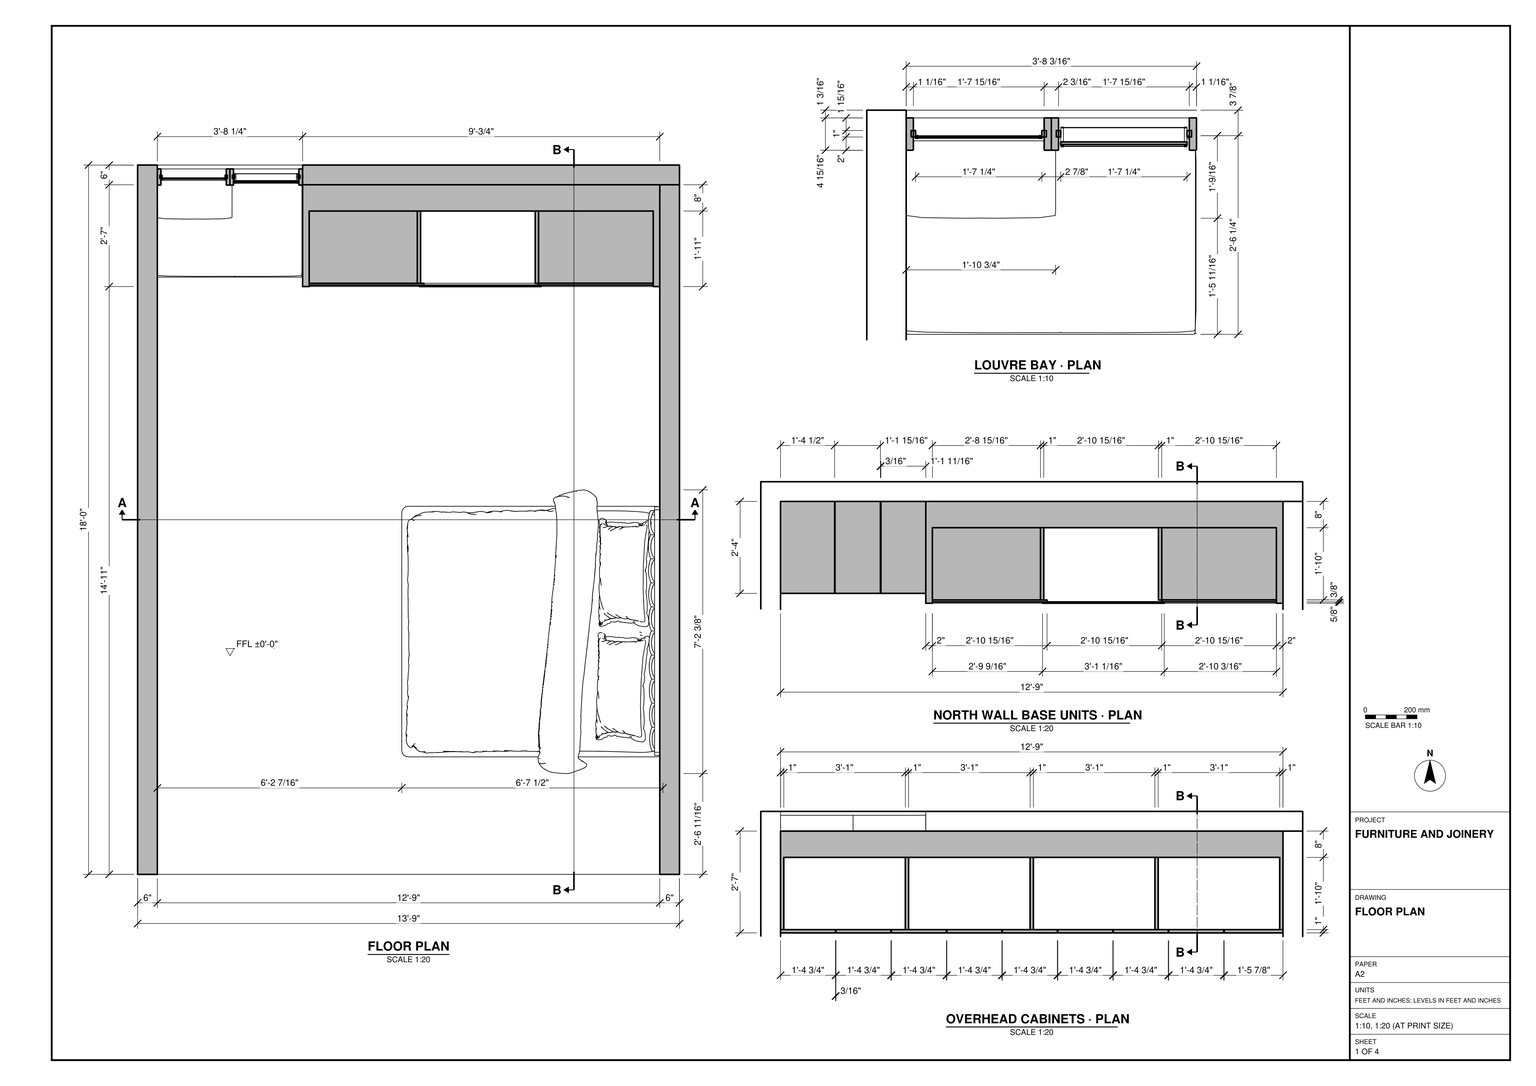
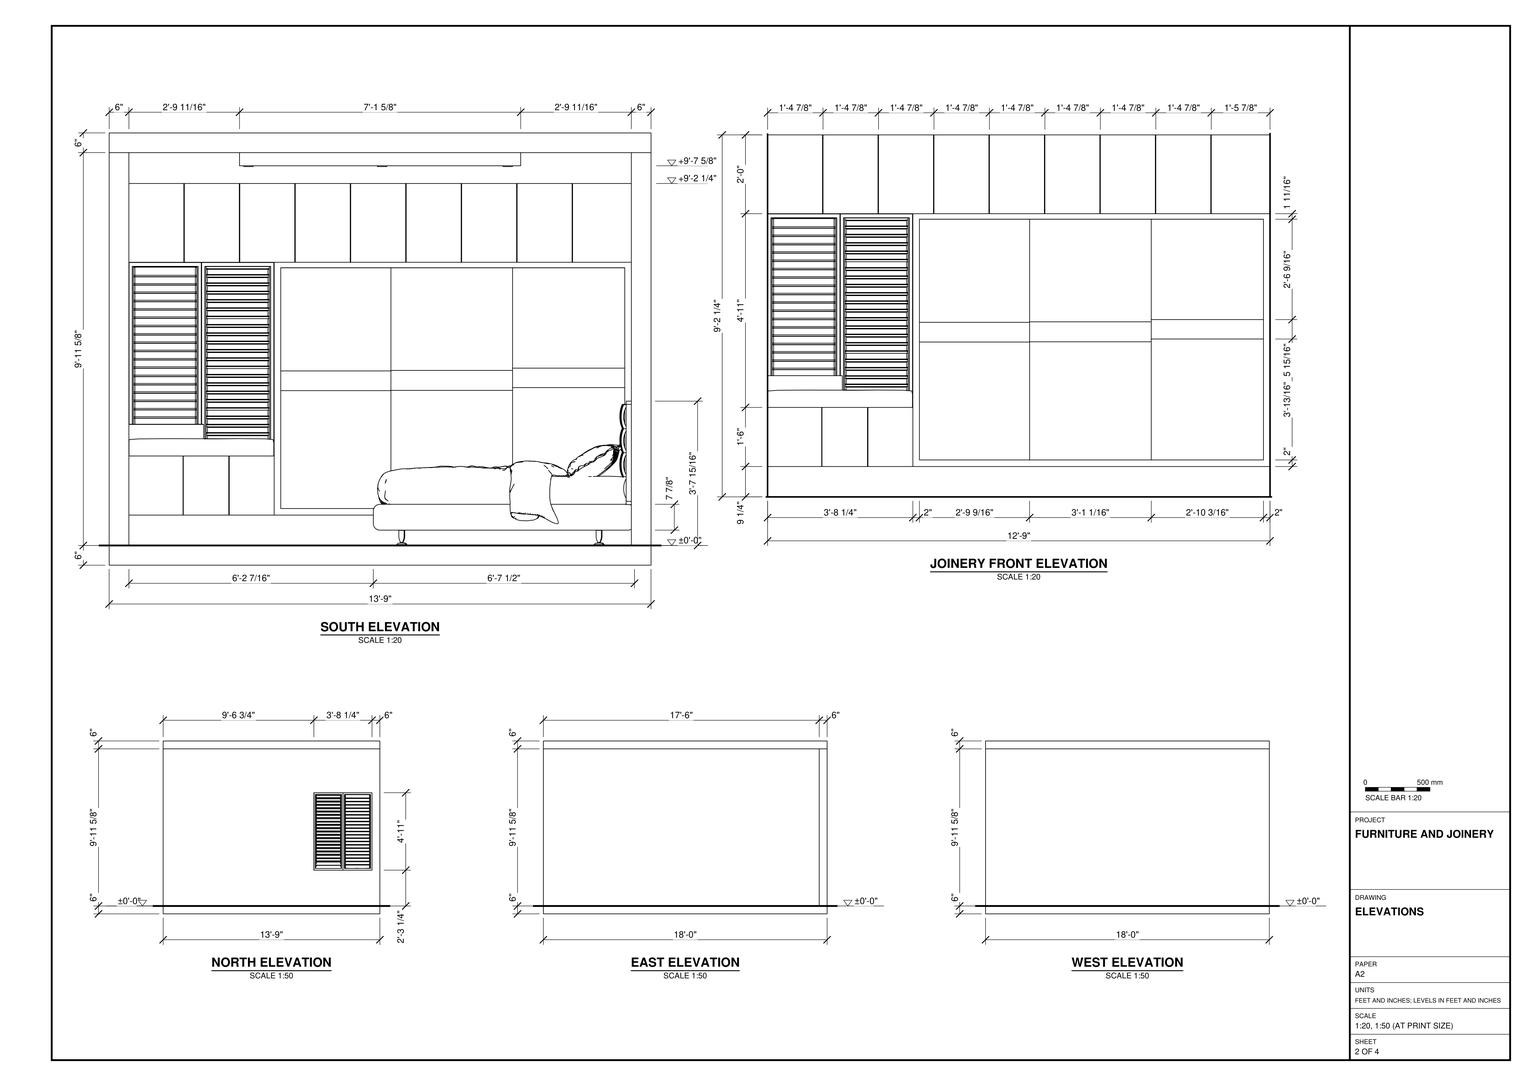
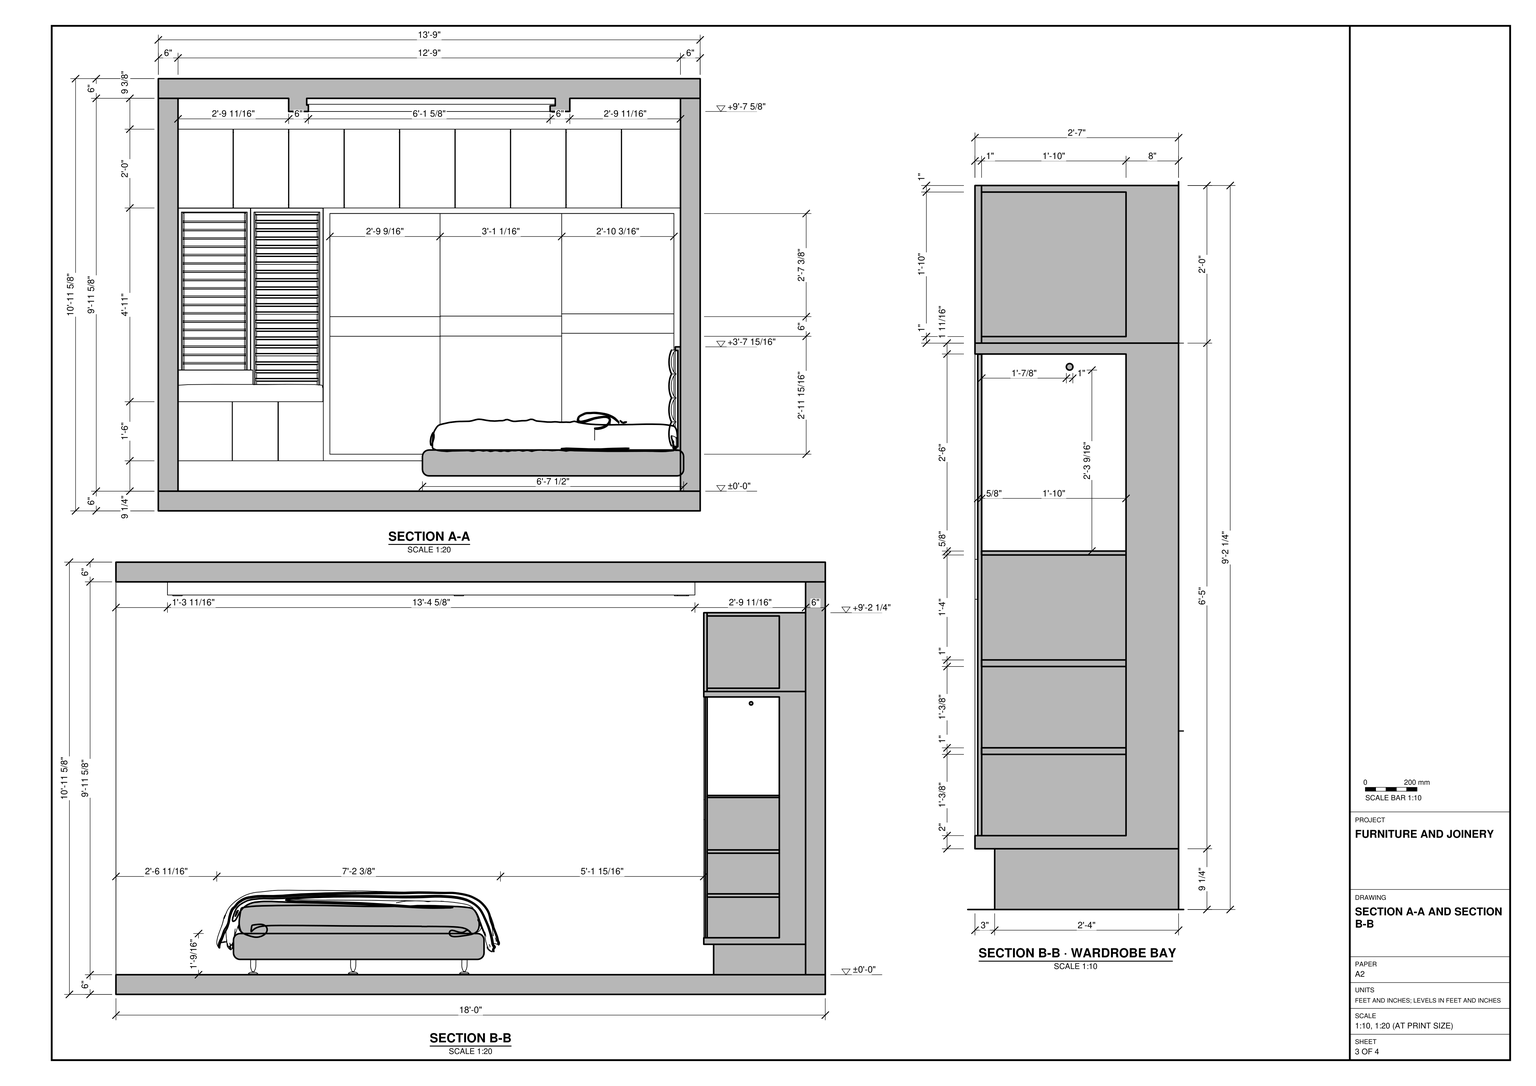
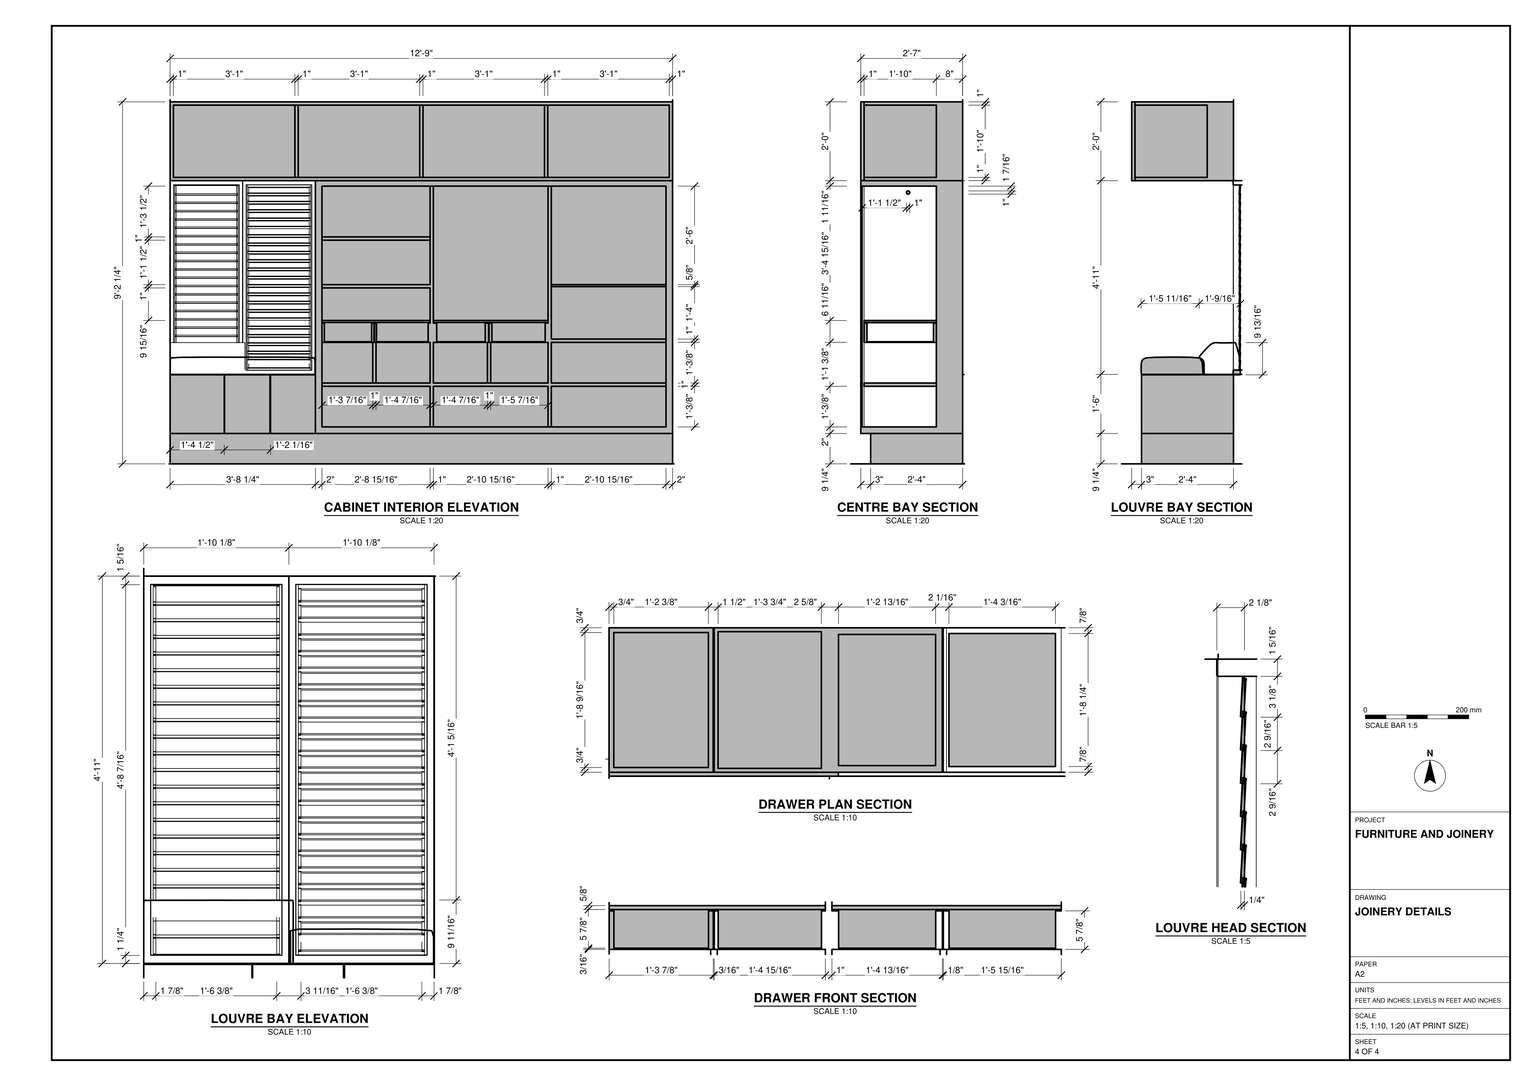
Model the bedroom in SketchUp using task_files/diagram_01.pdf. Work in feet and inches. Set the finished floor level to ±0'-0". The room shell measures 13'-9" east to west, 18'-0" north to south and 10'-11 5/8" high overall. Model the 6" side and north walls between the floor and ceiling slabs. Leave the south end open as drawn, and include the elongated ceiling feature shown in the sections.

Fit the joinery across the north wall. At the west end, place the two framed louvred window units above the sill and low cabinets. Beside them, model the three tall wardrobe bays with the front divisions shown in elevation. Use the wardrobe section to set out the recessed plinth, shelves and hanging rail. Continue the overhead cabinets across both the window bay and the wardrobes. Place the bed with its headboard against the east wall and its foot facing west, leaving the clearances shown in plan. Include the raised bed base, mattress and bedding.

Decor and loose items may be any suitable library components. Keep shell elements and each furniture or joinery piece in separate groups or components, and use components for repeated parts. Save one SketchUp model as output_files/bedroom_with_fitted_wardrobes_and_a_louvred_window.skp.

# SketchUp Ruby script. Lengths in inches.
U = 1.inch
M = Sketchup.active_model
def pt(a) = Geom::Point3d.new(a.map { |v| v * U })
def face(e, loops, mat)
  f = e.add_face(loops[0].map { |a| pt(a) })
  loops[1..].each { |l| e.add_face(l.map { |a| pt(a) }).erase! }
  f.material = f.back_material = mat if mat
  f
end
# faces: each face lists its corners as indices into pts; further lists are holes
def faces(e, pts, list, mat = nil) = list.each { |f| face(e, (f[0].is_a?(Array) ? f : [f]).map { |l| l.map { |i| pts[i] } }, mat) }
# xy, xz, yz: faces in a plane at the given z, y or x. An outline is a flat list of corners, or four numbers for a rectangle; further outlines are holes
def ring(l) = l.size == 4 ? [[l[0], l[1]], [l[2], l[1]], [l[2], l[3]], [l[0], l[3]]] : l.each_slice(2).to_a
def flat(e, list, mat, &to3) = list.each { |f| face(e, (f[0].is_a?(Array) ? f : [f]).map { |l| ring(l).map { |u, v| to3.(u, v) } }, mat) }
def xy(e, z, list, mat = nil) = flat(e, list, mat) { |x, y| [x, y, z] }
def xz(e, y, list, mat = nil) = flat(e, list, mat) { |x, z| [x, y, z] }
def yz(e, x, list, mat = nil) = flat(e, list, mat) { |y, z| [x, y, z] }
def lines(e, pts, list) = list.each { |a, b| e.add_line(pt(pts[a]), pt(pts[b])) }
# prism: a flat outline (further loops are holes) pulled along v
def prism(e, loops, v, mat = nil)
  f = face(e, loops, mat); d = Geom::Vector3d.new(v.map { |x| x * U })
  f.pushpull(f.normal.samedirection?(d) ? d.length : -d.length)
end
def box(e, o, s, mat = nil) = prism(e, [[o, [o[0] + s[0], o[1], o[2]], [o[0] + s[0], o[1] + s[1], o[2]], [o[0], o[1] + s[1], o[2]]]], [0, 0, s[2]], mat)
def at(x, y, z, deg = 0) = Geom::Transformation.translation(pt([x, y, z])) * Geom::Transformation.rotation(ORIGIN, Z_AXIS, deg.degrees)
def axes(o, x, y, z) = Geom::Transformation.new([*x, 0, *y, 0, *z, 0, *pt(o).to_a, 1])
def part(name) = M.definitions.add(name)
# library, detail: a bought-in or finely detailed component or shape, given as its bounding box
def library(name, o, s) = part(name).tap { |d| box(d.entities, o, s) }
def detail(e, o, s) = box(e.add_group.entities, o, s)
def put(e, d, t, mat = nil) = e.add_instance(d, t).tap { |i| i.material = mat if mat }
def group(e, t, mat = nil) = e.add_group.tap { |g| g.transformation = t; g.material = mat if mat }.entities
root = M.entities
M.materials.add("GLASS BLADE REFRACTION").color = [24, 24, 24]
M.materials["GLASS BLADE REFRACTION"].alpha = 0.5
M.materials.add("JalousieFrame").color = [89, 86, 86]
M.materials.add("[0002_MediumVioletRed]").color = [204, 196, 185]
M.materials.add("[0003_DeepPink]").color = [255, 20, 147]
M.materials.add("[Color A01]").color = [207, 198, 188]
M.materials.add("[Color A01]1").color = [135, 122, 106]
M.materials.add("[Color A01]2").color = [96, 100, 74]
M.materials.add("[Color A02]").color = [146, 166, 154]
M.materials.add("[Color A02]1").color = [177, 163, 128]
M.materials.add("[Color A03]").color = [255, 101, 101]
M.materials.add("[Color H05]").color = [0, 255, 255]
M.materials.add("[Color M00]").color = [255, 255, 255]
M.materials.add("[Metal Corrugated Shiny]").color = [193, 193, 193]
M.materials.add("[Tile Large Brown]").color = [195, 178, 159]
M.materials.add("[Translucent Glass Blue]").color = [100, 149, 237]
M.materials["[Translucent Glass Blue]"].alpha = 0.5
M.materials.add("[Translucent Glass Corrugated]").color = [141, 158, 145]
M.materials["[Translucent Glass Corrugated]"].alpha = 0.8
M.materials.add("[Translucent_Glass_Blue]1").color = [0, 0, 0]
M.materials["[Translucent_Glass_Blue]1"].alpha = 0
M.materials.add("[Wood OSB]").color = [240, 195, 122]
c1 = part("Louvre end clip")
prism(c1.entities,[[[0,0.74,4.2],[0,0.38,4.24],[0,-0.06,-0.03],[0,0.29,-0.06],[0,0.3125,0.17],[0,0.26,0.18],[0,0.24,-0.02],[0,-0.02,0.01],[0,0.42,4.2],[0,0.68,4.17],[0,0.66,3.97],[0,0.71,3.97]]],[-0.59,0,0],"JalousieFrame")
c2 = part("Louvre blade")
xy(c2.entities,0,[[3.2,0,48.34,0.24]],"GLASS BLADE REFRACTION")
xy(c2.entities,4.17,[[3.2,0,48.34,0.24]],"GLASS BLADE REFRACTION")
xz(c2.entities,0,[[3.2,0,48.34,4.17]],"[Translucent Glass Blue]")
xz(c2.entities,0.24,[[3.2,0,48.34,4.17]],"[Translucent_Glass_Blue]1")
yz(c2.entities,3.2,[[0,0,0.24,4.17]],"[Translucent_Glass_Blue]1")
yz(c2.entities,48.34,[[0,0,0.24,4.17]],"[Translucent_Glass_Blue]1")
c3 = part("Louvre blade assembly")
put(c3.entities,c1,axes([29.56,0.12,0.28],[1,0,0],[0,1.01433,-0.13582],[0,-0.20296,0.86161]))
put(c3.entities,c1,axes([1.96,0.12,0.28],[-1,0,0],[0,1.01433,-0.13582],[0,-0.20296,0.86161]))
put(c3.entities,c2,axes([0,0.12,0.3],[0.61176,0,0],[0,1.02999,-0.22514],[0,-0.09582,0.84269]))
c4 = part("Louvre blade assembly \#1")
put(c4.entities,c3,axes([-2.4,1.66,-0.39],[1.63462,0,0],[0,0.98741,-0.15853],[0,0.15779,0.98741]),"[Translucent Glass Corrugated]")
c5 = part("Group6\#2")
box(c5.entities,[-2.07,2.02,1.67],[0.98,0.98,67.72],"JalousieFrame")
c6 = part("Louvred window")
xz(c6.entities,3.09,[[2.06,1.67,29.07,69.26]])
put(c6.entities,c4,axes([1.57,0.98,65.83],[0.61176,0,0],[0,1,0],[0,0,0.99766]))
put(c6.entities,c4,axes([1.57,0.98,62.79],[0.61176,0,0],[0,1,0],[0,0,0.99766]))
put(c6.entities,c4,axes([1.57,0.98,59.75],[0.61176,0,0],[0,1,0],[0,0,0.99766]))
put(c6.entities,c4,axes([1.57,0.98,56.7],[0.61176,0,0],[0,1,0],[0,0,0.99766]))
put(c6.entities,c4,axes([1.57,0.98,53.66],[0.61176,0,0],[0,1,0],[0,0,0.99766]))
put(c6.entities,c4,axes([1.57,0.98,50.61],[0.61176,0,0],[0,1,0],[0,0,0.99766]))
put(c6.entities,c4,axes([1.57,0.98,47.57],[0.61176,0,0],[0,1,0],[0,0,0.99766]))
put(c6.entities,c4,axes([1.57,0.98,44.53],[0.61176,0,0],[0,1,0],[0,0,0.99766]))
put(c6.entities,c4,axes([1.57,0.98,41.48],[0.61176,0,0],[0,1,0],[0,0,0.99766]))
put(c6.entities,c4,axes([1.57,0.98,38.4375],[0.61176,0,0],[0,1,0],[0,0,0.99766]))
put(c6.entities,c4,axes([1.57,0.98,35.39],[0.61176,0,0],[0,1,0],[0,0,0.99766]))
put(c6.entities,c4,axes([1.57,0.98,32.35],[0.61176,0,0],[0,1,0],[0,0,0.99766]))
put(c6.entities,c4,axes([1.57,0.98,29.31],[0.61176,0,0],[0,1,0],[0,0,0.99766]))
put(c6.entities,c4,axes([1.57,0.98,26.26],[0.61176,0,0],[0,1,0],[0,0,0.99766]))
put(c6.entities,c4,axes([1.57,0.98,23.22],[0.61176,0,0],[0,1,0],[0,0,0.99766]))
put(c6.entities,c4,axes([1.57,0.98,20.17],[0.61176,0,0],[0,1,0],[0,0,0.99766]))
put(c6.entities,c4,axes([1.57,0.98,17.13],[0.61176,0,0],[0,1,0],[0,0,0.99766]))
put(c6.entities,c4,axes([1.57,0.98,14.09],[0.61176,0,0],[0,1,0],[0,0,0.99766]))
put(c6.entities,c4,axes([1.57,0.98,11.04],[0.61176,0,0],[0,1,0],[0,0,0.99766]))
put(c6.entities,c4,axes([1.57,0.98,8],[0.61176,0,0],[0,1,0],[0,0,0.99766]))
put(c6.entities,c4,axes([1.57,0.98,4.95],[0.61176,0,0],[0,1,0],[0,0,0.99766]))
put(c6.entities,c4,axes([1.57,0.98,1.91],[0.61176,0,0],[0,1,0],[0,0,0.99766]))
g1 = group(c6.entities,at(0,0.98,0.1))
xy(g1,0,[[0,0.1,31.72,4.92]],"JalousieFrame")
xy(g1,1.57,[[1.57,0.1,30.15,4.92]],"JalousieFrame")
xy(g1,69.29,[[1.57,0.1,30.15,4.92]],"JalousieFrame")
xy(g1,70.87,[[0,0.1,31.72,4.92]],"JalousieFrame")
xz(g1,0,[[[0.1,0.1,31.625,70.77],[1.47,1.48,30.25,69.39]]],"JalousieFrame")
xz(g1,4.92,[[[0,0,31.72,70.87],[1.57,1.57,30.15,69.29]]],"JalousieFrame")
yz(g1,0,[[0.1,0,4.92,70.87]],"JalousieFrame")
yz(g1,1.57,[[0.1,1.57,4.92,69.29]],"JalousieFrame")
yz(g1,30.15,[[0.1,1.57,4.92,69.29]],"JalousieFrame")
yz(g1,31.72,[[0.1,0,4.92,70.87]],"JalousieFrame")
p = [[0,0.1,70.87],[0,0.1,0],[0.1,0,0.1],[0.1,0,70.77],[31.72,0.1,0],[31.625,0,0.1],
  [31.72,0.1,70.87],[31.625,0,70.77],[30.15,0.1,1.57],[1.57,0.1,1.57],[1.47,0,1.48],[30.25,0,1.48],
  [1.57,0.1,69.29],[1.47,0,69.39],[30.15,0.1,69.29],[30.25,0,69.39]]
faces(g1,p,[[0,1,2,3],[1,4,5,2],[4,6,7,5],[8,9,10,11],[9,12,13,10],[14,8,11,15],[12,14,15,13],[6,0,3,7]],"JalousieFrame")
put(c6.entities,c5,axes([31.72,0.98,0],[0.99482,0,0],[0,1,0],[0,0,1]))
put(c6.entities,c5,axes([0,0.98,0],[-0.99482,0,0],[0,1,0],[0,0,1]))
c7 = part("Louvre blade assembly \#2")
put(c7.entities,c3,axes([-2.4,0.24,0.625],[1.63462,0,0],[0,0.5,-0.86805],[0,0.864,0.5]))
c8 = part("Group6\#1")
box(c8.entities,[-2.07,2.02,1.67],[0.98,0.98,67.72],"JalousieFrame")
c9 = part("Louvred window \#1")
put(c9.entities,c7,axes([1.57,0.98,65.83],[0.61176,0,0],[0,1,0],[0,0,0.99766]))
put(c9.entities,c7,axes([1.57,0.98,62.79],[0.61176,0,0],[0,1,0],[0,0,0.99766]))
put(c9.entities,c7,axes([1.57,0.98,59.75],[0.61176,0,0],[0,1,0],[0,0,0.99766]))
put(c9.entities,c7,axes([1.57,0.98,56.7],[0.61176,0,0],[0,1,0],[0,0,0.99766]))
put(c9.entities,c7,axes([1.57,0.98,53.66],[0.61176,0,0],[0,1,0],[0,0,0.99766]))
put(c9.entities,c7,axes([1.57,0.98,50.61],[0.61176,0,0],[0,1,0],[0,0,0.99766]))
put(c9.entities,c7,axes([1.57,0.98,47.57],[0.61176,0,0],[0,1,0],[0,0,0.99766]))
put(c9.entities,c7,axes([1.57,0.98,44.53],[0.61176,0,0],[0,1,0],[0,0,0.99766]))
put(c9.entities,c7,axes([1.57,0.98,41.48],[0.61176,0,0],[0,1,0],[0,0,0.99766]))
put(c9.entities,c7,axes([1.57,0.98,38.4375],[0.61176,0,0],[0,1,0],[0,0,0.99766]))
put(c9.entities,c7,axes([1.57,0.98,35.39],[0.61176,0,0],[0,1,0],[0,0,0.99766]))
put(c9.entities,c7,axes([1.57,0.98,32.35],[0.61176,0,0],[0,1,0],[0,0,0.99766]))
put(c9.entities,c7,axes([1.57,0.98,29.31],[0.61176,0,0],[0,1,0],[0,0,0.99766]))
put(c9.entities,c7,axes([1.57,0.98,26.26],[0.61176,0,0],[0,1,0],[0,0,0.99766]))
put(c9.entities,c7,axes([1.57,0.98,23.22],[0.61176,0,0],[0,1,0],[0,0,0.99766]))
put(c9.entities,c7,axes([1.57,0.98,20.17],[0.61176,0,0],[0,1,0],[0,0,0.99766]))
put(c9.entities,c7,axes([1.57,0.98,17.13],[0.61176,0,0],[0,1,0],[0,0,0.99766]))
put(c9.entities,c7,axes([1.57,0.98,14.09],[0.61176,0,0],[0,1,0],[0,0,0.99766]))
put(c9.entities,c7,axes([1.57,0.98,11.04],[0.61176,0,0],[0,1,0],[0,0,0.99766]))
put(c9.entities,c7,axes([1.57,0.98,8],[0.61176,0,0],[0,1,0],[0,0,0.99766]))
put(c9.entities,c7,axes([1.57,0.98,4.95],[0.61176,0,0],[0,1,0],[0,0,0.99766]))
put(c9.entities,c7,axes([1.57,0.98,1.91],[0.61176,0,0],[0,1,0],[0,0,0.99766]))
g2 = group(c9.entities,at(0,0.98,0.1))
xy(g2,0,[[0,0.1,31.72,4.92]],"JalousieFrame")
xy(g2,1.57,[[1.57,0.1,30.15,4.92]],"JalousieFrame")
xy(g2,69.29,[[1.57,0.1,30.15,4.92]],"JalousieFrame")
xy(g2,70.87,[[0,0.1,31.72,4.92]],"JalousieFrame")
xz(g2,0,[[[0.1,0.1,31.625,70.77],[1.47,1.48,30.25,69.39]]],"JalousieFrame")
xz(g2,4.92,[[[0,0,31.72,70.87],[1.57,1.57,30.15,69.29]]],"JalousieFrame")
yz(g2,0,[[0.1,0,4.92,70.87]],"JalousieFrame")
yz(g2,1.57,[[0.1,1.57,4.92,69.29]],"JalousieFrame")
yz(g2,30.15,[[0.1,1.57,4.92,69.29]],"JalousieFrame")
yz(g2,31.72,[[0.1,0,4.92,70.87]],"JalousieFrame")
p = [[0,0.1,70.87],[0,0.1,0],[0.1,0,0.1],[0.1,0,70.77],[31.72,0.1,0],[31.625,0,0.1],
  [31.72,0.1,70.87],[31.625,0,70.77],[30.15,0.1,1.57],[1.57,0.1,1.57],[1.47,0,1.48],[30.25,0,1.48],
  [1.57,0.1,69.29],[1.47,0,69.39],[30.15,0.1,69.29],[30.25,0,69.39]]
faces(g2,p,[[0,1,2,3],[1,4,5,2],[4,6,7,5],[8,9,10,11],[9,12,13,10],[14,8,11,15],[12,14,15,13],[6,0,3,7]],"JalousieFrame")
put(c9.entities,c8,axes([31.72,0.98,0],[0.99482,0,0],[0,1,0],[0,0,1]))
put(c9.entities,c8,axes([0,0.98,0],[-0.99482,0,0],[0,1,0],[0,0,1]))
c10 = part("JSilva Jalousie")
put(c10.entities,c6,axes([-10.84,-0.98,0.02],[-0.66344,0,0],[0,1,0],[0,0,0.83238]))
put(c10.entities,c9,axes([10.2,-0.98,0.02],[-0.66344,0,0],[0,1,0],[0,0,0.83238]))
c11 = library("Natuzzi-Forma-2818-373",[-24.875,-9.99,1.67],[57.88,39.07,27.9])
c12 = part("Round vent grille")
xy(c12.entities,-0.25,[[[1.4375,0,1.07,0.05,0.72,0.19,0.42,0.42,0.19,0.72,0.05,1.07,0,1.4375,0.05,1.81,0.19,2.16,0.42,2.45,0.72,2.68,1.07,2.83,1.4375,2.875,1.81,2.83,2.16,2.68,2.45,2.45,2.68,2.16,2.83,1.81,2.875,1.4375,2.83,1.07,2.68,0.72,2.45,0.42,2.16,0.19,1.81,0.05],[1.4375,0.47,1.6875,0.51,1.92,0.6,2.12,0.76,2.27,0.96,2.37,1.1875,2.4,1.4375,2.37,1.6875,2.27,1.92,2.12,2.12,1.92,2.27,1.6875,2.37,1.4375,2.4,1.1875,2.37,0.96,2.27,0.76,2.12,0.6,1.92,0.51,1.6875,0.47,1.4375,0.51,1.1875,0.6,0.96,0.76,0.76,0.96,0.6,1.1875,0.51]]])
xy(c12.entities,-0.0625,[[1.4375,0.47,1.1875,0.51,0.96,0.6,0.76,0.76,0.6,0.96,0.51,1.1875,0.47,1.4375,0.51,1.6875,0.6,1.92,0.76,2.12,0.96,2.27,1.1875,2.37,1.4375,2.4,1.6875,2.37,1.92,2.27,2.12,2.12,2.27,1.92,2.37,1.6875,2.4,1.4375,2.37,1.1875,2.27,0.96,2.12,0.76,1.92,0.6,1.6875,0.51]])
xy(c12.entities,0,[[1.4375,0,1.81,0.05,2.16,0.19,2.45,0.42,2.68,0.72,2.83,1.07,2.875,1.4375,2.83,1.81,2.68,2.16,2.45,2.45,2.16,2.68,1.81,2.83,1.4375,2.875,1.07,2.83,0.72,2.68,0.42,2.45,0.19,2.16,0.05,1.81,0,1.4375,0.05,1.07,0.19,0.72,0.42,0.42,0.72,0.19,1.07,0.05]])
p = [[1.07,0.05,0],[0.72,0.19,0],[0.72,0.19,-0.25],[1.07,0.05,-0.25],[1.4375,0,0],[1.4375,0,-0.25],
  [1.81,0.05,0],[1.81,0.05,-0.25],[2.16,0.19,0],[2.16,0.19,-0.25],[0.42,0.42,0],[0.42,0.42,-0.25],
  [2.45,0.42,0],[2.45,0.42,-0.25],[0.19,0.72,0],[0.19,0.72,-0.25],[2.68,0.72,0],[2.68,0.72,-0.25],
  [1.1875,0.51,-0.25],[0.96,0.6,-0.25],[0.96,0.6,-0.0625],[1.1875,0.51,-0.0625],[1.4375,0.47,-0.25],[1.4375,0.47,-0.0625],
  [1.6875,0.51,-0.25],[1.6875,0.51,-0.0625],[1.92,0.6,-0.25],[1.92,0.6,-0.0625],[0.76,0.76,-0.25],[0.76,0.76,-0.0625],
  [2.12,0.76,-0.25],[2.12,0.76,-0.0625],[0.05,1.07,0],[0.05,1.07,-0.25],[2.83,1.07,0],[2.83,1.07,-0.25],
  [0.6,0.96,-0.25],[0.6,0.96,-0.0625],[2.27,0.96,-0.25],[2.27,0.96,-0.0625],[0.51,1.1875,-0.25],[0.51,1.1875,-0.0625],
  [2.37,1.1875,-0.25],[2.37,1.1875,-0.0625],[0,1.4375,0],[0,1.4375,-0.25],[2.875,1.4375,0],[2.875,1.4375,-0.25],
  [0.47,1.4375,-0.25],[0.47,1.4375,-0.0625],[2.4,1.4375,-0.25],[2.4,1.4375,-0.0625],[0.05,1.81,0],[0.05,1.81,-0.25],
  [0.51,1.6875,-0.25],[0.51,1.6875,-0.0625],[2.37,1.6875,-0.25],[2.37,1.6875,-0.0625],[2.83,1.81,0],[2.83,1.81,-0.25],
  [0.6,1.92,-0.25],[0.6,1.92,-0.0625],[2.27,1.92,-0.25],[2.27,1.92,-0.0625],[0.19,2.16,0],[0.19,2.16,-0.25],
  [2.68,2.16,0],[2.68,2.16,-0.25],[0.76,2.12,-0.25],[0.76,2.12,-0.0625],[2.12,2.12,-0.25],[2.12,2.12,-0.0625],
  [0.96,2.27,-0.25],[0.96,2.27,-0.0625],[1.92,2.27,-0.25],[1.92,2.27,-0.0625],[0.42,2.45,0],[0.42,2.45,-0.25],
  [2.45,2.45,0],[2.45,2.45,-0.25],[1.1875,2.37,-0.25],[1.1875,2.37,-0.0625],[1.6875,2.37,-0.25],[1.6875,2.37,-0.0625],
  [1.4375,2.4,-0.25],[1.4375,2.4,-0.0625],[0.72,2.68,0],[0.72,2.68,-0.25],[2.16,2.68,0],[2.16,2.68,-0.25],
  [1.07,2.83,0],[1.07,2.83,-0.25],[1.81,2.83,0],[1.81,2.83,-0.25],[1.4375,2.875,0],[1.4375,2.875,-0.25]]
faces(c12.entities,p,[[0,1,2,3],[4,0,3,5],[6,4,5,7],[8,6,7,9],[1,10,11,2],[12,8,9,13],[10,14,15,11],[16,12,13,17],
  [18,19,20,21],[22,18,21,23],[24,22,23,25],[26,24,25,27],[19,28,29,20],[30,26,27,31],[14,32,33,15],[34,16,17,35],
  [28,36,37,29],[38,30,31,39],[36,40,41,37],[42,38,39,43],[32,44,45,33],[46,34,35,47],[40,48,49,41],[50,42,43,51],
  [44,52,53,45],[48,54,55,49],[56,50,51,57],[58,46,47,59],[54,60,61,55],[62,56,57,63],[52,64,65,53],[66,58,59,67],
  [60,68,69,61],[70,62,63,71],[68,72,73,69],[74,70,71,75],[64,76,77,65],[78,66,67,79],[72,80,81,73],[82,74,75,83],
  [80,84,85,81],[84,82,83,85],[76,86,87,77],[88,78,79,89],[86,90,91,87],[92,88,89,93],[90,94,95,91],[94,92,93,95]])
c13 = library("master bed",[77.89,-32.24,0],[86.39,79.53,43.7])
c14 = part("Union")
xy(c14.entities,0,[[0,-1,108.76,30]],"[Color A01]")
xy(c14.entities,2,[[2,-1,106.76,22]],"[Color A01]")
xy(c14.entities,75.33,[[2,-1,106.76,22]],"[Color A01]")
xy(c14.entities,76.99,[[0,-1,108.76,0],[-44.24,0,0,30]],"[Color A01]")
xy(c14.entities,77.99,[[-43.24,0,107.76,22]],"[Color A01]")
xy(c14.entities,99.99,[[-43.24,0,107.76,22]],"[Color A01]")
xy(c14.entities,100.99,[[-44.24,0,108.76,30]],"[Color A01]")
xz(c14.entities,-1,[[[0,0,108.76,76.99],[2,2,106.76,75.33]]],"[Color A01]")
xz(c14.entities,0,[[[-44.24,76.99,108.76,100.99],[-43.24,77.99,107.76,99.99]]],"[Color A01]")
xz(c14.entities,22,[[2,2,106.76,75.33],[-43.24,77.99,107.76,99.99]],"[Color A01]")
xz(c14.entities,30,[[0,0,0,76.99,-44.24,76.99,-44.24,100.99,108.76,100.99,108.76,0]],"[Color A01]")
yz(c14.entities,-44.24,[[0,76.99,30,100.99]],"[Color A01]")
yz(c14.entities,-43.24,[[0,77.99,22,99.99]],"[Color A01]")
yz(c14.entities,0,[[-1,0,30,76.99]],"[Color A01]")
yz(c14.entities,2,[[-1,2,22,75.33]],"[Color A01]")
yz(c14.entities,106.76,[[-1,2,22,75.33]],"[Color A01]")
yz(c14.entities,107.76,[[0,77.99,22,99.99]],"[Color A01]")
yz(c14.entities,108.76,[[-1,0,30,0,30,100.99,0,100.99,0,76.99,-1,76.99]],"[Color A01]")
c15 = part("Group\#6")
box(c15.entities,[-1,0,0],[1,22,22])
c16 = part("Group\#9")
box(c16.entities,[-1,0,0],[1,22,12.38])
c17 = part("Union\#2")
box(c17.entities,[0,0,0],[34.92,22,0.6])
c18 = part("Union\#1")
box(c18.entities,[0,0,0],[32.92,22,0.6])
c19 = part("Union\#3")
box(c19.entities,[-2,0,0],[34.92,22,0.6])
xy(root,11.25,[[85.16,180,86.16,202],[121.08,180,122.08,202]])
xy(root,23.62,[[52.24,180,85.16,202],[86.16,180,121.08,202],[122.08,180,157,202]])
xy(root,24.62,[[52.24,180,85.16,202],[86.16,180,121.08,202],[122.08,180,157,202]])
xy(root,37,[[52.24,180,68.09,202],[68.25,180,68.7,202],[68.7,180,85.16,202],[86.16,180,102.62,202],[102.62,180,102.98,202],
  [103.12,180,121.08,202],[122.08,180,157,202]])
xy(root,37.1875,[[68.84,180.59,84.57,201.41],[52.97,180.73,67.37,201.27],[103.99,180.87,120.21,201.13],[87.18,181.02,101.96,200.98]])
xy(root,38,[[122.08,180,157,202]])
xy(root,41.28,[[57.85,180,59.98,180.1875],[74.91,180,77.04,180.1875],[92.91,180,95.04,180.1875],[110.6,180,112.73,180.1875]],"[0002_MediumVioletRed]")
xy(root,41.71,[[57.85,180,59.98,180.1875],[74.91,180,77.04,180.1875],[92.91,180,95.04,180.1875],[110.6,180,112.73,180.1875]],"[0002_MediumVioletRed]")
xy(root,42.86,[[[52.24,180,68.09,202],[52.97,180.73,67.37,201.27]],[[68.25,180,85.16,202],[68.84,180.59,84.57,201.41]],[[86.16,180,102.98,202],[87.18,181.02,101.96,200.98]],[[103.12,180,121.08,202],[103.99,180.87,120.21,201.13]]])
xy(root,53.58,[[52.24,180,85.16,202]])
xy(root,54.58,[[52.24,180,85.16,202]])
xy(root,84.55,[[85.16,180,86.16,202],[121.08,180,122.08,202]])
xz(root,180,[[85.16,11.25,86.16,11.25,86.16,23.62,121.08,23.62,121.08,11.25,122.08,11.25,122.08,23.62,157,23.62,157,24.62,122.08,24.62,122.08,37,157,37,157,37.02,121.08,37.02,121.08,24.62,86.16,24.62,86.16,84.55,85.16,84.55,85.16,24.62,52.24,24.62,52.24,23.62,85.16,23.62],[[52.24,37,68.09,42.86],[57.74,41.17,60.08,41.82]],[[68.25,37,85.16,42.86],[74.81,41.17,77.15,41.82]],[[86.16,37,102.98,42.86],[92.81,41.17,95.15,41.82]],[[103.12,37,121.08,42.86],[110.49,41.17,112.83,41.82]],
  [121.08,37.02,157,37.02,157,38,122.08,38,122.08,84.55,121.08,84.55],[52.24,53.58,85.16,54.58]])
xz(root,180,[[[57.74,41.17,60.08,41.82],[57.85,41.28,59.98,41.71]],[[74.81,41.17,77.15,41.82],[74.91,41.28,77.04,41.71]],[[92.81,41.17,95.15,41.82],[92.91,41.28,95.04,41.71]],[[110.49,41.17,112.83,41.82],[110.6,41.28,112.73,41.71]]],"[Wood OSB]")
xz(root,180.1875,[[57.85,41.28,59.98,41.71],[74.91,41.28,77.04,41.71],[92.91,41.28,95.04,41.71],[110.6,41.28,112.73,41.71]],"[0002_MediumVioletRed]")
xz(root,180.59,[[68.84,37.1875,84.57,42.86]])
xz(root,180.73,[[52.97,37.1875,67.37,42.86]])
xz(root,180.87,[[103.99,37.1875,120.21,42.86]])
xz(root,181.02,[[87.18,37.1875,101.96,42.86]])
xz(root,200.98,[[87.18,37.1875,101.96,42.86]])
xz(root,201.13,[[103.99,37.1875,120.21,42.86]])
xz(root,201.27,[[52.97,37.1875,67.37,42.86]])
xz(root,201.41,[[68.84,37.1875,84.57,42.86]])
xz(root,202,[[85.16,11.25,85.16,23.62,52.24,23.62,52.24,24.62,85.16,24.62,85.16,37,68.25,37,68.25,42.86,85.16,42.86,85.16,53.58,52.24,53.58,52.24,54.58,85.16,54.58,85.16,84.55,86.16,84.55,86.16,42.86,102.98,42.86,102.98,37,86.16,37,86.16,24.62,121.08,24.62,121.08,37,103.12,37,103.12,42.86,121.08,42.86,121.08,84.55,122.08,84.55,122.08,38,157,38,157,37,122.08,37,122.08,24.62,157,24.62,157,23.62,122.08,23.62,122.08,11.25,121.08,11.25,121.08,23.62,86.16,23.62,86.16,11.25],[52.24,37,68.09,42.86],[68.09,37,68.25,43.0625],[102.98,37,103.12,37.0625]])
yz(root,52.24,[[180,23.62,202,24.62],[180,37,202,42.86],[180,53.58,202,54.58]])
yz(root,52.97,[[180.73,37.1875,201.27,42.86]])
yz(root,57.85,[[180,41.28,180.1875,41.71]],"[0002_MediumVioletRed]")
yz(root,59.98,[[180,41.28,180.1875,41.71]])
yz(root,67.37,[[180.73,37.1875,201.27,42.86]])
yz(root,68.09,[[180,37,202,37.0625],[180,37.0625,202,42.86]])
yz(root,68.25,[[180,37,202,37.0625],[180,37.0625,202,42.86]])
yz(root,68.84,[[180.59,37.1875,201.41,42.86]])
yz(root,74.91,[[180,41.28,180.1875,41.71]],"[0002_MediumVioletRed]")
yz(root,77.04,[[180,41.28,180.1875,41.71]],"[0002_MediumVioletRed]")
yz(root,84.57,[[180.59,37.1875,201.41,42.86]])
yz(root,85.16,[[180,11.25,202,23.62],[180,24.62,202,37],[180,42.86,202,53.58],[180,54.58,202,84.55]])
yz(root,86.16,[[180,11.25,202,23.62],[180,24.62,202,37],[180,42.86,202,84.55]])
yz(root,87.18,[[181.02,37.1875,200.98,42.86]])
yz(root,92.91,[[180,41.28,180.1875,41.71]],"[0002_MediumVioletRed]")
yz(root,95.04,[[180,41.28,180.1875,41.71]],"[0002_MediumVioletRed]")
yz(root,101.96,[[181.02,37.1875,200.98,42.86]])
yz(root,102.98,[[180,37,202,42.86]])
yz(root,103.12,[[180,37,202,42.86]])
yz(root,103.99,[[180.87,37.1875,201.13,42.86]])
yz(root,110.6,[[180,41.28,180.1875,41.71]],"[0003_DeepPink]")
yz(root,112.73,[[180,41.28,180.1875,41.71]],"[0002_MediumVioletRed]")
yz(root,120.21,[[180.87,37.1875,201.13,42.86]])
yz(root,121.08,[[180,11.25,202,23.62],[180,24.62,202,37],[180,42.86,202,84.55]])
yz(root,122.08,[[180,11.25,202,23.62],[180,24.62,202,37],[180,38,202,84.55]])
yz(root,157,[[180,23.62,202,24.62],[180,37,202,38]])
p = [[85.79,179.4,53.16],[86.16,179.4,53.16],[85.79,179.4,47.16],[86.16,179.4,47.16]]
lines(root,p,[[0,1],[2,3]])
put(root,c10,axes([39.48,209.9,27.15],[1.05,0,0],[0,1,0],[0,0,1]))
put(root,c11,axes([24.97,189.6,26.53],[0.76243,0,0],[0,0.77414,0],[0,0,0.3515]))
put(root,c12,at(40.99,17.3,115.625))
put(root,c12,at(81.67,17.3,115.625))
put(root,c12,at(119.92,17.3,115.625))
put(root,c12,at(40.99,102.99,115.625))
put(root,c12,at(119.92,102.99,115.625))
put(root,c12,at(81.67,171.55,115.625))
put(root,c12,at(119.92,170.99,115.625))
put(root,c12,at(40.99,170.05,115.625))
put(root,c13,at(112.66,194.98,0.25,-90))
g3 = group(root,at(0,-24,0),"[Color A01]")
xy(g3,0,[[0,24,0,240,165,240,165,234,6,234,6,24]])
xy(g3,27.25,[[6,234,50.24,240]])
xy(g3,86.24,[[6,234,50.24,240]])
xy(g3,119.625,[[0,24,6,24,6,234,165,234,165,240,0,240]])
xz(g3,24,[[0,0,6,119.625]])
xz(g3,234,[[6,0,165,0,165,119.625,6,119.625,6,86.24,50.24,86.24,50.24,27.25,6,27.25]])
xz(g3,240,[[[0,0,165,119.625],[6,27.25,50.24,86.24]]])
yz(g3,0,[[24,0,240,119.625]])
yz(g3,6,[[24,0,234,0,234,27.25,240,27.25,240,86.24,234,86.24,234,119.625,24,119.625]])
yz(g3,50.24,[[234,27.25,240,86.24]])
yz(g3,165,[[234,0,240,119.625]])
g4 = group(root,at(159,-24,0),"[Color A01]")
xy(g4,0,[[0,24,6,234]])
xy(g4,119.625,[[0,24,6,234]])
xz(g4,24,[[0,0,6,119.625]])
xz(g4,234,[[0,0,6,119.625]])
yz(g4,0,[[24,0,234,119.625]],"[Color A01]2")
yz(g4,6,[[24,0,234,119.625]])
g5 = group(root,at(6,-24,0),"[Color A01]")
xy(g5,-6,[[-6,24,159,240]])
xy(g5,0,[[-6,24,159,240]],"[Tile Large Brown]")
xz(g5,24,[[-6,-6,159,0]])
xz(g5,240,[[-6,-6,159,0]])
yz(g5,-6,[[24,-6,240,0]])
yz(g5,159,[[24,-6,240,0]])
g6 = group(root,at(6,-24,125.625))
xy(g6,-10,[[[33.69,39.69,119.31,200.31],[39.69,45.69,113.31,194.31]]],"[Color H05]")
xy(g6,-8.375,[[39.69,44.07,113.31,45.69]],"[Color H05]")
xy(g6,-8.25,[[113.31,44.07,114.87,194.31]],"[Color H05]")
xy(g6,-8.0625,[[39.19,44.07,39.69,194.31]],"[Color H05]")
xy(g6,-7.8125,[[39.19,194.31,114.87,196.49]])
xy(g6,-6,[[[-6,24,159,240],[33.69,39.69,119.31,200.31]]])
xy(g6,-6,[[39.19,44.07,114.87,196.49]],"[Color M00]")
xy(g6,0,[[-6,24,159,240]])
xz(g6,24,[[-6,-6,159,0]])
xz(g6,39.69,[[33.69,-10,119.31,-6]],"[Color H05]")
xz(g6,44.07,[[39.69,-8.375,39.69,-8.0625,39.19,-8.0625,39.19,-6,114.87,-6,114.87,-8.25,113.31,-8.25,113.31,-8.375]],"[Color A03]")
xz(g6,45.69,[[39.69,-10,113.31,-8.375]],"[Color H05]")
xz(g6,194.31,[[39.69,-10,113.31,-10,113.31,-8.25,114.87,-8.25,114.87,-7.8125,39.19,-7.8125,39.19,-8.0625,39.69,-8.0625]],"[Color H05]")
xz(g6,196.49,[[39.19,-7.8125,114.87,-6]],"[Color A03]")
xz(g6,200.31,[[33.69,-10,119.31,-6]])
xz(g6,240,[[-6,-6,159,0]])
yz(g6,-6,[[24,-6,240,0]])
yz(g6,33.69,[[39.69,-10,200.31,-6]],"[Color H05]")
yz(g6,39.19,[[44.07,-8.0625,194.31,-8.0625,194.31,-7.8125,196.49,-7.8125,196.49,-6,44.07,-6]],"[Color A03]")
yz(g6,39.69,[[45.69,-10,194.31,-10,194.31,-8.0625,44.07,-8.0625,44.07,-8.375,45.69,-8.375]],"[Color H05]")
yz(g6,113.31,[[45.69,-10,45.69,-8.375,44.07,-8.375,44.07,-8.25,194.31,-8.25,194.31,-10]],"[Color H05]")
yz(g6,114.87,[[44.07,-8.25,44.07,-6,196.49,-6,196.49,-7.8125,194.31,-7.8125,194.31,-8.25]],"[Color A03]")
yz(g6,119.31,[[39.69,-10,200.31,-6]],"[Color H05]")
yz(g6,159,[[24,-6,240,0]])
p = [[113.31,196.49,-8.25],[113.31,194.31,-8.25],[114.87,45.69,-8.375],[113.31,45.69,-8.375],[39.69,45.69,-8.375],[39.19,45.69,-8.375]]
lines(g6,p,[[0,1],[2,3],[4,5]])
g7 = group(root,at(50.24,180,0))
prism(g7,[[[-44.24,2,0],[108.76,2,0],[108.76,2,9.25],[0,2,9.25],[-44.24,2,9.25]]],[0,28,0],"[Color A01]")
p = [[0,2,9.25],[0,0,9.25]]
lines(g7,p,[[0,1]])
put(root,c14,at(50.24,180,9.25))
g8 = group(root,at(50.24,180,86.24))
xy(g8,0,[[0,0,108.76,30]])
put(root,c15,at(45,180,87.24))
put(root,c15,at(83,180,87.24))
put(root,c15,at(121,180,87.24))
g9 = group(root,at(6,179,86.24),"[Color A01]")
box(g9,[16.89,0,0],[16.73,1,24])
box(g9,[33.78,0,0],[16.73,1,24])
box(g9,[0,0,0],[16.73,1,24])
box(g9,[118.22,0,0],[16.73,1,24])
box(g9,[101.33,0,0],[16.73,1,24])
box(g9,[50.67,0,0],[16.73,1,24])
box(g9,[67.56,0,0],[16.73,1,24])
box(g9,[84.44,0,0],[16.74,1,24])
box(g9,[135.11,0,0],[17.89,1,24])
g10 = group(root,at(52.24,180,68.11))
box(g10,[0,0,0],[32.92,22,1])
put(root,c16,at(103.62,180,24.62))
put(root,c16,at(68.7,180,24.62))
put(root,c17,at(86.16,180,43.0625))
put(root,c18,at(52.24,180,43.0625))
put(root,c19,at(124.08,180,53.98))
g11 = group(root,at(86.16,192.91,82.13))
prism(g11,[[[0,0,0.5625],[0,0.03,0.6875],[0,0.1,0.8],[0,0.19,0.89],[0,0.31,0.96],[0,0.43,0.99],[0,0.5625,0.99],[0,0.6875,0.96],[0,0.8,0.89],[0,0.89,0.8],[0,0.96,0.69],[0,0.99,0.56],[0,0.99,0.43],[0,0.96,0.3],[0,0.89,0.19],[0,0.8,0.1],[0,0.69,0.03],[0,0.56,0],[0,0.43,0],[0,0.3,0.03],[0,0.19,0.1],[0,0.1,0.19],[0,0.03,0.31],[0,0,0.43]]],[34.92,0,0],"[Metal Corrugated Shiny]")
p = [[0,0.54,0.51],[34.92,0.54,0.51]]
lines(g11,p,[[0,1]])
g12 = group(root,at(122.08,192.91,82.13),"[Metal Corrugated Shiny]")
prism(g12,[[[0,0,0.5625],[0,0.03,0.6875],[0,0.1,0.8],[0,0.19,0.89],[0,0.31,0.96],[0,0.43,0.99],[0,0.5625,0.99],[0,0.6875,0.96],[0,0.8,0.89],[0,0.89,0.8],[0,0.96,0.69],[0,0.99,0.56],[0,0.99,0.43],[0,0.96,0.3],[0,0.89,0.19],[0,0.8,0.1],[0,0.69,0.03],[0,0.56,0],[0,0.43,0],[0,0.3,0.03],[0,0.19,0.1],[0,0.1,0.19],[0,0.03,0.31],[0,0,0.43]]],[34.92,0,0],"[Metal Corrugated Shiny]")
p = [[0,0.54,0.51],[34.92,0.54,0.51]]
lines(g12,p,[[0,1]])
g13 = group(root,at(6,180,9.25))
box(g13,[30.57,2,0],[13.67,28,18],"[Color A01]")
box(g13,[16.58,2,0],[13.83,28,18],"[Color A01]")
box(g13,[0,2,0],[16.48,28,18],"[Color A01]")
p = [[16.48,30,0],[16.58,30,0],[44.24,2,0],[44.24,0,0],[30.41,30,0],[30.57,30,0]]
lines(g13,p,[[0,1],[2,3],[4,5]])
g14 = group(root,at(52.24,179,11.25))
g15 = group(g14,at(0,1,26.75))
xy(g15,-26.75,[[0,-0.6,34.92,0]])
xy(g15,46.55,[[0,-0.6,34.92,0]])
xz(g15,-0.6,[[0,9.16,34.92,15.16]])
xz(g15,-0.6,[[0,-26.75,34.92,9.16]],"[Color A01]1")
xz(g15,-0.6,[[0,15.16,34.92,46.55]],"[Color A02]")
xz(g15,0,[[0,-26.75,34.92,46.55]])
yz(g15,0,[[-0.6,-26.75,0,46.55]])
yz(g15,34.92,[[-0.6,-26.75,0,46.55]])
g16 = group(g14,at(33.55,0.4,26.75))
xy(g16,-26.75,[[0,-0.4,37.05,0]])
xy(g16,46.55,[[0,-0.4,37.05,0]])
xz(g16,-0.4,[[0,9.23,37.05,15.3125]])
xz(g16,-0.4,[[0,-26.75,37.05,9.23]],"[Color A02]")
xz(g16,-0.4,[[0,15.3125,37.05,46.55]],"[Color A02]1")
xz(g16,0,[[0,-26.75,37.05,46.55]])
yz(g16,0,[[-0.4,9.23,0,15.3125]])
yz(g16,0,[[-0.4,-26.75,0,9.23]],"[Color A02]")
yz(g16,0,[[-0.4,15.3125,0,46.55]],"[Color A02]1")
yz(g16,37.05,[[-0.4,9.23,0,15.3125]])
yz(g16,37.05,[[-0.4,-26.75,0,9.23]],"[Color A02]")
yz(g16,37.05,[[-0.4,15.3125,0,46.55]],"[Color A02]1")
g17 = group(g14,at(69.84,1.02,26.75))
xy(g17,-26.75,[[0,-0.6,34.92,0]])
xy(g17,46.55,[[0,-0.6,34.92,0]])
xz(g17,-0.6,[[0,10.08,34.92,16]])
xz(g17,-0.6,[[0,16,34.92,46.55]],"[Color A01]1")
xz(g17,-0.6,[[0,-26.75,34.92,10.08]],"[Color A02]1")
xz(g17,0,[[0,-26.75,34.92,46.55]])
yz(g17,0,[[-0.6,-26.75,0,10.08],[-0.6,10.08,0,16],[-0.6,16,0,46.55]])
yz(g17,34.92,[[-0.6,-26.75,0,10.08],[-0.6,10.08,0,16],[-0.6,16,0,46.55]])
p = [[34.92,0,15.23],[34.92,0.03,15.23]]
lines(g17,p,[[0,1]])
